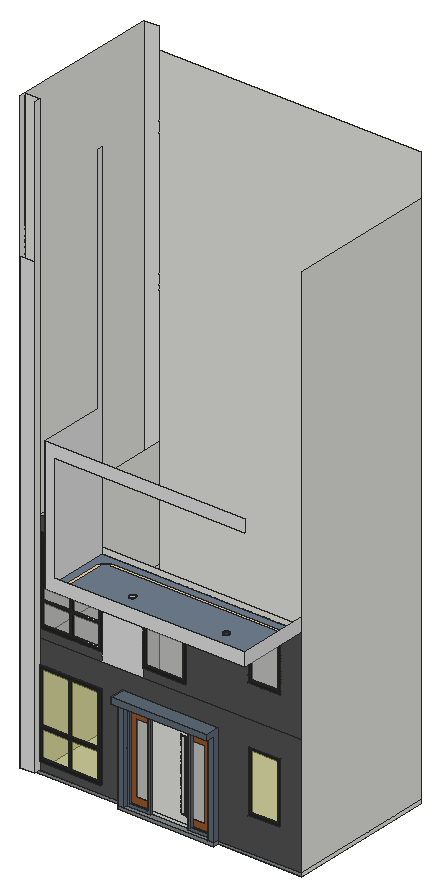
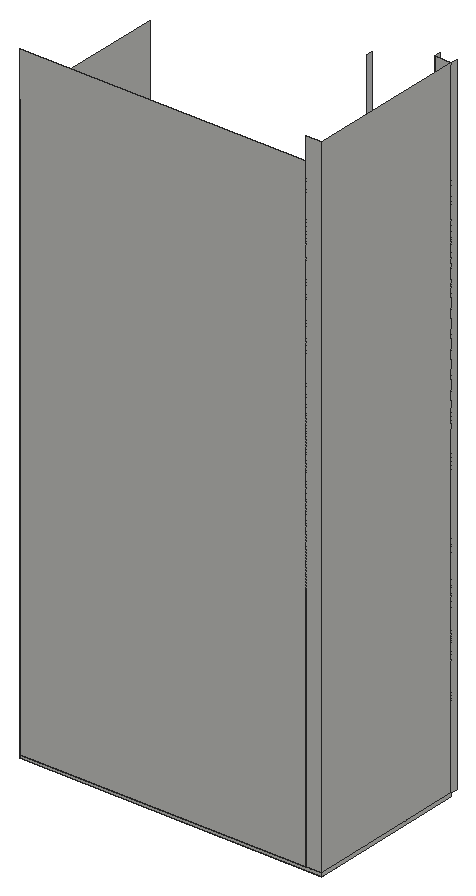
# SketchUp Ruby script. Lengths in inches.
U = 1.inch
M = Sketchup.active_model
def pt(a) = Geom::Point3d.new(a.map { |v| v * U })
def face(e, loops, mat)
  f = e.add_face(loops[0].map { |a| pt(a) })
  loops[1..].each { |l| e.add_face(l.map { |a| pt(a) }).erase! }
  f.material = f.back_material = mat if mat
  f
end
# faces: each face lists its corners as indices into pts; further lists are holes
def faces(e, pts, list, mat = nil) = list.each { |f| face(e, (f[0].is_a?(Array) ? f : [f]).map { |l| l.map { |i| pts[i] } }, mat) }
# xy, xz, yz: faces in a plane at the given z, y or x. An outline is a flat list of corners, or four numbers for a rectangle; further outlines are holes
def ring(l) = l.size == 4 ? [[l[0], l[1]], [l[2], l[1]], [l[2], l[3]], [l[0], l[3]]] : l.each_slice(2).to_a
def flat(e, list, mat, &to3) = list.each { |f| face(e, (f[0].is_a?(Array) ? f : [f]).map { |l| ring(l).map { |u, v| to3.(u, v) } }, mat) }
def xy(e, z, list, mat = nil) = flat(e, list, mat) { |x, y| [x, y, z] }
def xz(e, y, list, mat = nil) = flat(e, list, mat) { |x, z| [x, y, z] }
def yz(e, x, list, mat = nil) = flat(e, list, mat) { |y, z| [x, y, z] }
def lines(e, pts, list) = list.each { |a, b| e.add_line(pt(pts[a]), pt(pts[b])) }
# prism: a flat outline (further loops are holes) pulled along v
def prism(e, loops, v, mat = nil)
  f = face(e, loops, mat); d = Geom::Vector3d.new(v.map { |x| x * U })
  f.pushpull(f.normal.samedirection?(d) ? d.length : -d.length)
end
def box(e, o, s, mat = nil) = prism(e, [[o, [o[0] + s[0], o[1], o[2]], [o[0] + s[0], o[1] + s[1], o[2]], [o[0], o[1] + s[1], o[2]]]], [0, 0, s[2]], mat)
def at(x, y, z, deg = 0) = Geom::Transformation.translation(pt([x, y, z])) * Geom::Transformation.rotation(ORIGIN, Z_AXIS, deg.degrees)
def axes(o, x, y, z) = Geom::Transformation.new([*x, 0, *y, 0, *z, 0, *pt(o).to_a, 1])
def part(name) = M.definitions.add(name)
# library, detail: a bought-in or finely detailed component or shape, given as its bounding box
def library(name, o, s) = part(name).tap { |d| box(d.entities, o, s) }
def detail(e, o, s) = box(e.add_group.entities, o, s)
def put(e, d, t, mat = nil) = e.add_instance(d, t).tap { |i| i.material = mat if mat }
def group(e, t, mat = nil) = e.add_group.tap { |g| g.transformation = t; g.material = mat if mat }.entities
root = M.entities
M.materials.add("[0033_NavajoWhite]1").color = [237, 206, 160]
M.materials.add("[0110_LightSlateGray]").color = [93, 106, 119]
M.materials.add("[0111_SlateGray]").color = [112, 128, 144]
M.materials.add("[0132_LightGray]").color = [102, 102, 102]
M.materials.add("[0136_Charcoal]").color = [35, 35, 35]
M.materials.add("[Blacktop Old 01]").color = [132, 136, 139]
M.materials.add("[Cladding Siding White]1").color = [224, 224, 224]
M.materials.add("[Cladding Siding White]2").color = [81, 81, 81]
M.materials.add("[Translucent Glass Gray]1").color = [163, 163, 163]
M.materials["[Translucent Glass Gray]1"].alpha = 0.5
M.materials.add("[Translucent Glass Gray]2").color = [204, 203, 94]
M.materials["[Translucent Glass Gray]2"].alpha = 0.5
M.materials.add("[Translucent Glass Gray]3").color = [130, 130, 130]
M.materials["[Translucent Glass Gray]3"].alpha = 0.5
M.materials.add("[Wood Cherry Original]").color = [152, 86, 42]
xy(root,0,[[396,264,396,288,0,288,0,888,1116,888,1116,288,780,288,780,264]])
xy(root,12,[[0,264,60,288],[396,264,416.85,288],[759.15,264,780,288],[416.85,281,511.85,288],[664.15,281,759.15,288],
  [0,288,60,888],[60,288,1116,888]])
xy(root,12,[[416.85,264,759.15,264,759.15,281,664.15,281,664.15,288,511.85,288,511.85,281,416.85,281]],"[Blacktop Old 01]")
xy(root,23,[[427.85,281,499.85,288],[676.15,281,748.15,288]],"[0110_LightSlateGray]")
xy(root,48,[[60,282,312,288]],"[0136_Charcoal]")
xy(root,59.16,[[634.86,288,648.92,294]])
xy(root,60,[[72,282,181,288],[191,282,300,288]],"[0136_Charcoal]")
xy(root,156,[[912,288,1020,294]],"[0136_Charcoal]")
xy(root,168,[[72,282,181,288],[191,282,300,288]],"[0136_Charcoal]")
xy(root,180,[[72,282,181,288],[191,282,300,288]],"[0136_Charcoal]")
xy(root,338.39,[[634.86,288,648.92,294]])
xy(root,364.15,[[427.85,281,499.85,288],[511.85,281,664.15,288],[676.15,281,748.15,288]],"[0110_LightSlateGray]")
xy(root,375.15,[[416.85,281,759.15,288]])
xy(root,375.15,[[416.85,264,759.15,281]],"[0110_LightSlateGray]")
xy(root,384,[[181,282,191,288]])
xy(root,384,[[72,282,181,288],[191,282,300,288],[912,288,1020,294]],"[0136_Charcoal]")
xy(root,396,[[396,228,780,264]],"[0110_LightSlateGray]")
xy(root,396,[[60,282,312,288]],"[0136_Charcoal]")
xy(root,420,[[396,228,780,288]],"[0110_LightSlateGray]")
xy(root,540,[[72,288,181,295],[191,288,300,295]])
xy(root,540,[[487.9375,288,636,294]],"[0136_Charcoal]")
xy(root,624,[[72,288,181,295],[191,288,300,295]],"[0136_Charcoal]")
xy(root,630,[[72,288,181,295],[191,288,300,295]])
xy(root,636,[[912,288,1020,294]],"[0136_Charcoal]")
xy(root,864,[[72,288,181,295],[191,288,300,295],[487.9375,288,636,294],[912,288,1020,294]],"[0136_Charcoal]")
xy(root,882.9375,[[[385.0625,34.5,380.03,34.83,375.08,35.8125,370.3,37.43,365.78,39.67,361.59,42.47,357.79,45.79,354.47,49.59,351.67,53.78,349.43,58.3,347.8125,63.08,346.83,68.03,346.5,73.0625,346.5,214.9375,346.83,219.97,347.8125,224.92,349.43,229.7,351.67,234.22,354.47,238.41,357.79,242.21,361.59,245.53,365.78,248.33,370.3,250.57,375.08,252.1875,380.03,253.17,385.0625,253.5,1042.9375,253.5,1047.97,253.17,1052.92,252.1875,1057.7,250.57,1062.22,248.33,1066.41,245.53,1070.21,242.21,1073.53,238.41,1076.33,234.22,1078.57,229.7,1080.1875,224.92,1081.17,219.97,1081.5,214.9375,1081.5,73.0625,1081.17,68.03,1080.1875,63.08,1078.57,58.3,1076.33,53.78,1073.53,49.59,1070.21,45.79,1066.41,42.47,1062.22,39.67,1057.7,37.43,1052.92,35.8125,1047.97,34.83,1042.9375,34.5],[385.0625,40.83,1042.9375,40.83,1047.15,41.11,1051.28,41.93,1055.27,43.29,1059.05,45.15,1062.56,47.49,1065.73,50.27,1068.51,53.44,1070.85,56.95,1072.71,60.73,1074.07,64.72,1074.89,68.85,1075.17,73.0625,1075.17,214.9375,1074.89,219.15,1074.07,223.28,1072.71,227.27,1070.85,231.05,1068.51,234.56,1065.73,237.73,1062.56,240.51,1059.05,242.85,1055.27,244.71,1051.28,246.07,1047.15,246.89,1042.9375,247.17,385.0625,247.17,380.85,246.89,376.72,246.07,372.73,244.71,368.95,242.85,365.44,240.51,362.27,237.73,359.49,234.56,357.15,231.05,355.29,227.27,353.93,223.28,353.11,219.15,352.83,214.9375,352.83,73.0625,353.11,68.85,353.93,64.72,355.29,60.73,357.15,56.95,359.49,53.44,362.27,50.27,365.44,47.49,368.95,45.15,372.73,43.29,376.72,41.93,380.85,41.11]]],"[0033_NavajoWhite]1")
xy(root,882.9375,[[[312,0,1116,288],[385.0625,34.5,1042.9375,34.5,1047.97,34.83,1052.92,35.8125,1057.7,37.43,1062.22,39.67,1066.41,42.47,1070.21,45.79,1073.53,49.59,1076.33,53.78,1078.57,58.3,1080.1875,63.08,1081.17,68.03,1081.5,73.0625,1081.5,214.9375,1081.17,219.97,1080.1875,224.92,1078.57,229.7,1076.33,234.22,1073.53,238.41,1070.21,242.21,1066.41,245.53,1062.22,248.33,1057.7,250.57,1052.92,252.1875,1047.97,253.17,1042.9375,253.5,385.0625,253.5,380.03,253.17,375.08,252.1875,370.3,250.57,365.78,248.33,361.59,245.53,357.79,242.21,354.47,238.41,351.67,234.22,349.43,229.7,347.8125,224.92,346.83,219.97,346.5,214.9375,346.5,73.0625,346.83,68.03,347.8125,63.08,349.43,58.3,351.67,53.78,354.47,49.59,357.79,45.79,361.59,42.47,365.78,39.67,370.3,37.43,375.08,35.8125,380.03,34.83]],[[385.0625,40.83,380.85,41.11,376.72,41.93,372.73,43.29,368.95,45.15,365.44,47.49,362.27,50.27,359.49,53.44,357.15,56.95,355.29,60.73,353.93,64.72,353.11,68.85,352.83,73.0625,352.83,214.9375,353.11,219.15,353.93,223.28,355.29,227.27,357.15,231.05,359.49,234.56,362.27,237.73,365.44,240.51,368.95,242.85,372.73,244.71,376.72,246.07,380.85,246.89,385.0625,247.17,1042.9375,247.17,1047.15,246.89,1051.28,246.07,1055.27,244.71,1059.05,242.85,1062.56,240.51,1065.73,237.73,1068.51,234.56,1070.85,231.05,1072.71,227.27,1074.07,223.28,1074.89,219.15,1075.17,214.9375,1075.17,73.0625,1074.89,68.85,1074.07,64.72,1072.71,60.73,1070.85,56.95,1068.51,53.44,1065.73,50.27,1062.56,47.49,1059.05,45.15,1055.27,43.29,1051.28,41.93,1047.15,41.11,1042.9375,40.83],[559.63,120.38,560.88,120.5,562.11,120.75,563.31,121.13,564.46,121.63,565.55,122.25,566.57,122.98,567.51,123.82,568.36,124.74,569.11,125.76,569.74,126.84,570.26,127.98,570.66,129.17,570.93,130.4,571.07,131.65,571.08,132.9,570.96,134.15,570.71,135.39,570.33,136.58,569.82,137.73,569.2,138.83,568.47,139.85,567.64,140.79,566.71,141.64,565.7,142.38,564.62,143.02,563.48,143.54,562.28,143.93,561.06,144.2,559.81,144.35,558.55,144.35,557.3,144.23,556.07,143.98,554.875,143.6,553.72,143.1,552.63,142.48,551.61,141.75,550.67,140.92,549.82,139.99,549.08,138.98,548.44,137.9,547.92,136.75,547.52,135.56,547.25,134.33,547.11,133.09,547.1,131.83,547.23,130.58,547.48,129.35,547.86,128.15,548.36,127,548.98,125.91,549.71,124.89,550.54,123.95,551.47,123.1,552.48,122.35,553.5625,121.72,554.71,121.2,555.9,120.8,557.125,120.53,558.375,120.39],[937.5,120.38,938.75,120.5,939.98,120.75,941.18,121.13,942.33,121.63,943.43,122.25,944.45,122.98,945.39,123.82,946.24,124.74,946.98,125.76,947.62,126.84,948.14,127.98,948.53,129.17,948.8,130.4,948.95,131.65,948.95,132.9,948.83,134.15,948.58,135.39,948.2,136.58,947.7,137.73,947.08,138.83,946.35,139.85,945.52,140.79,944.59,141.64,943.58,142.38,942.5,143.02,941.35,143.54,940.16,143.93,938.93,144.2,937.69,144.35,936.43,144.35,935.18,144.23,933.95,143.98,932.75,143.6,931.6,143.1,930.51,142.48,929.49,141.75,928.55,140.92,927.7,139.99,926.95,138.98,926.32,137.9,925.8,136.75,925.4,135.56,925.13,134.33,924.99,133.09,924.98,131.83,925.1,130.58,925.35,129.35,925.73,128.15,926.23,127,926.85,125.91,927.58,124.89,928.42,123.95,929.34,123.1,930.36,122.35,931.4375,121.72,932.58,121.2,933.77,120.8,935,120.53,936.25,120.39]]],"[0111_SlateGray]")
xz(root,0,[[312,882.9375,1116,882.9375,1116,936,348,936,348,1366.34,1116,1366.34,1116,1416,312,1416]],"[Cladding Siding White]1")
xz(root,144.35,[[558.55,882.9375,559.81,883.9375],[936.43,882.9375,937.69,883.9375]])
xz(root,228,[[396,396,780,420]],"[0110_LightSlateGray]")
xz(root,264,[[396,12,416.85,12,416.85,375.15,759.15,375.15,759.15,12,780,12,780,396,396,396]],"[0110_LightSlateGray]")
xz(root,264,[[396,0,780,12]],"[Blacktop Old 01]")
xz(root,264,[[0,12,60,1858.15]],"[Cladding Siding White]1")
xz(root,281,[[[416.85,12,511.85,12,511.85,364.15,664.15,364.15,664.15,12,759.15,12,759.15,375.15,416.85,375.15],[427.85,23,499.85,364.15],[676.15,23,748.15,364.15]]],"[0110_LightSlateGray]")
xz(root,282,[[[60,48,312,396],[72,180,72,384,300,384,300,180,191,180,191,384,181,384,181,180],[191,60,300,168],[72,60,181,168]]],"[0136_Charcoal]")
xz(root,288,[[0,12,60,2436],[396,12,396,396,780,396,780,12,759.15,12,759.15,375.15,416.85,375.15,416.85,12],[[416.85,12,416.85,375.15,759.15,375.15,759.15,12,664.15,12,664.15,364.15,511.85,364.15,511.85,12],[427.85,23,499.85,364.15],[676.15,23,748.15,364.15]],[511.85,12,664.15,23],[[511.85,23,664.15,364.15],[628.7,53,655.08,344.55]],
  [[60,48,312,396],[72,180,181,180,181,384,191,384,191,180,300,180,300,384,72,384],[191,60,300,168],[72,60,181,168]],[312,882.9375,1116,906]])
xz(root,288,[[[628.7,53,655.08,344.55],[634.86,59.16,648.92,338.39]]],"[0132_LightGray]")
xz(root,288,[[[900,144,1032,396],[912,156,1020,384]],[[60,528,312,876],[191,630,300,864],[72,630,181,864],[72,540,181,624],[191,540,300,624]],[[475.9375,528,648,876],[487.9375,540,636,864]],[[900,624,1032,876],[912,636,1020,864]]],"[0136_Charcoal]")
xz(root,288,[[0,0,396,12],[780,0,1116,12]],"[Blacktop Old 01]")
xz(root,288,[[312,492,475.9375,882.9375]],"[Cladding Siding White]1")
xz(root,288,[[[60,12,396,12,396,420,780,420,780,12,1116,12,1116,492,60,492,60,396,312,396,312,48,60,48],[900,144,1032,396]],[60,492,312,528],[[475.9375,492,1116,492,1116,882.9375,475.9375,882.9375,475.9375,876,648,876,648,528,475.9375,528],[900,624,1032,876]],[60,876,312,936]],"[Cladding Siding White]2")
xz(root,288,[[72,60,181,168],[191,60,300,168],[72,180,181,384],[191,180,300,384]],"[Translucent Glass Gray]2")
xz(root,288,[[451.85,53,499.85,334.15],[676.15,53,724.15,334.15]],"[Translucent Glass Gray]3")
xz(root,288,[[427.85,23,499.85,23,499.85,53,451.85,53,451.85,334.15,499.85,334.15,499.85,364.15,427.85,364.15],[676.15,23,748.15,23,748.15,364.15,676.15,364.15,676.15,334.15,724.15,334.15,724.15,53,676.15,53]],"[Wood Cherry Original]")
xz(root,294,[[634.86,59.16,648.92,338.39]],"[0132_LightGray]")
xz(root,294,[[487.9375,540,636,864],[912,636,1020,864]],"[Translucent Glass Gray]1")
xz(root,294,[[912,156,1020,384]],"[Translucent Glass Gray]2")
xz(root,295,[[72,540,181,624],[191,540,300,624],[72,630,181,864],[191,630,300,864]],"[Translucent Glass Gray]1")
xz(root,888,[[0,0,1116,12],[0,12,60,2436],[60,12,1116,2352]])
yz(root,0,[[288,0,888,12],[264,12,288,2436],[288,12,888,2436]])
yz(root,60,[[264,12,288,12,288,48,282,48,282,396,288,396,288,2436,264,2436],[288,12,888,492],[282,48,288,396],[288,492,888,936]])
yz(root,72,[[282,60,288,168],[282,180,288,384],[288,540,295,624],[288,630,295,864]],"[0136_Charcoal]")
yz(root,181,[[288,540,295,624],[288,630,295,864]])
yz(root,181,[[282,60,288,168],[282,180,288,384]],"[0136_Charcoal]")
yz(root,191,[[282,60,288,168],[282,180,288,384],[288,540,295,624],[288,630,295,864]],"[0136_Charcoal]")
yz(root,300,[[282,60,288,168],[282,180,288,384],[288,540,295,624],[288,630,295,864]],"[0136_Charcoal]")
yz(root,312,[[282,48,288,396]],"[0136_Charcoal]")
yz(root,312,[[0,882.9375,0,1416,264,1416,264,2352,288,2352,288,882.9375]],"[Cladding Siding White]1")
yz(root,396,[[264,12,264,396,228,396,228,420,288,420,288,12]],"[0110_LightSlateGray]")
yz(root,396,[[264,0,288,12]],"[Blacktop Old 01]")
yz(root,416.85,[[281,12,288,375.15]])
yz(root,416.85,[[264,12,281,375.15]],"[0110_LightSlateGray]")
yz(root,427.85,[[281,23,288,364.15]],"[0110_LightSlateGray]")
yz(root,487.9375,[[288,540,294,864]],"[0136_Charcoal]")
yz(root,499.85,[[281,23,288,364.15]],"[0110_LightSlateGray]")
yz(root,511.85,[[281,12,288,364.15]],"[0110_LightSlateGray]")
yz(root,634.86,[[288,59.16,294,338.39]])
yz(root,636,[[288,540,294,864]],"[0136_Charcoal]")
yz(root,648.92,[[288,59.16,294,338.39]])
yz(root,664.15,[[281,12,288,364.15]],"[0110_LightSlateGray]")
yz(root,676.15,[[281,23,288,364.15]],"[0110_LightSlateGray]")
yz(root,748.15,[[281,23,288,364.15]],"[0110_LightSlateGray]")
yz(root,759.15,[[281,12,288,375.15]])
yz(root,759.15,[[264,12,281,375.15]],"[0110_LightSlateGray]")
yz(root,780,[[264,12,288,12,288,420,228,420,228,396,264,396]],"[0110_LightSlateGray]")
yz(root,780,[[264,0,288,12]],"[Blacktop Old 01]")
yz(root,912,[[288,156,294,384],[288,636,294,864]],"[0136_Charcoal]")
yz(root,948.95,[[131.65,882.9375,132.9,883.9375]])
yz(root,1020,[[288,156,294,384],[288,636,294,864]],"[0136_Charcoal]")
yz(root,1116,[[288,0,888,12],[288,12,888,2184]])
yz(root,1116,[[0,882.9375,288,936]],"[Cladding Siding White]1")
p = [[558.375,120.39,882.9375],[557.125,120.53,882.9375],[557.125,120.53,883.9375],[558.375,120.39,883.9375],[559.63,120.38,882.9375],[559.63,120.38,883.9375],
  [560.88,120.5,882.9375],[560.88,120.5,883.9375],[936.25,120.39,882.9375],[935,120.53,882.9375],[935,120.53,883.9375],[936.25,120.39,883.9375],
  [937.5,120.38,882.9375],[937.5,120.38,883.9375],[938.75,120.5,882.9375],[938.75,120.5,883.9375],[555.9,120.8,882.9375],[555.9,120.8,883.9375],
  [562.11,120.75,882.9375],[562.11,120.75,883.9375],[933.77,120.8,882.9375],[933.77,120.8,883.9375],[939.98,120.75,882.9375],[939.98,120.75,883.9375],
  [554.71,121.2,882.9375],[554.71,121.2,883.9375],[563.31,121.13,882.9375],[563.31,121.13,883.9375],[932.58,121.2,882.9375],[932.58,121.2,883.9375],
  [941.18,121.13,882.9375],[941.18,121.13,883.9375],[564.46,121.63,882.9375],[564.46,121.63,883.9375],[942.33,121.63,882.9375],[942.33,121.63,883.9375],
  [553.5625,121.72,882.9375],[553.5625,121.72,883.9375],[931.4375,121.72,882.9375],[931.4375,121.72,883.9375],[565.55,122.25,882.9375],[565.55,122.25,883.9375],
  [943.43,122.25,882.9375],[943.43,122.25,883.9375],[552.48,122.35,882.9375],[552.48,122.35,883.9375],[930.36,122.35,882.9375],[930.36,122.35,883.9375],
  [566.57,122.98,882.9375],[566.57,122.98,883.9375],[944.45,122.98,882.9375],[944.45,122.98,883.9375],[551.47,123.1,882.9375],[551.47,123.1,883.9375],
  [929.34,123.1,882.9375],[929.34,123.1,883.9375],[567.51,123.82,882.9375],[567.51,123.82,883.9375],[945.39,123.82,882.9375],[945.39,123.82,883.9375],
  [550.54,123.95,882.9375],[550.54,123.95,883.9375],[928.42,123.95,882.9375],[928.42,123.95,883.9375],[568.36,124.74,882.9375],[568.36,124.74,883.9375],
  [946.24,124.74,882.9375],[946.24,124.74,883.9375],[549.71,124.89,882.9375],[549.71,124.89,883.9375],[927.58,124.89,882.9375],[927.58,124.89,883.9375],
  [569.11,125.76,882.9375],[569.11,125.76,883.9375],[946.98,125.76,882.9375],[946.98,125.76,883.9375],[548.98,125.91,882.9375],[548.98,125.91,883.9375],
  [926.85,125.91,882.9375],[926.85,125.91,883.9375],[569.74,126.84,882.9375],[569.74,126.84,883.9375],[947.62,126.84,882.9375],[947.62,126.84,883.9375],
  [548.36,127,882.9375],[548.36,127,883.9375],[926.23,127,882.9375],[926.23,127,883.9375],[570.26,127.98,882.9375],[570.26,127.98,883.9375],
  [948.14,127.98,882.9375],[948.14,127.98,883.9375],[547.86,128.15,882.9375],[547.86,128.15,883.9375],[925.73,128.15,882.9375],[925.73,128.15,883.9375],
  [570.66,129.17,882.9375],[570.66,129.17,883.9375],[948.53,129.17,882.9375],[948.53,129.17,883.9375],[547.48,129.35,882.9375],[547.48,129.35,883.9375],
  [925.35,129.35,882.9375],[925.35,129.35,883.9375],[570.93,130.4,882.9375],[570.93,130.4,883.9375],[948.8,130.4,882.9375],[948.8,130.4,883.9375],
  [547.23,130.58,882.9375],[547.23,130.58,883.9375],[925.1,130.58,882.9375],[925.1,130.58,883.9375],[571.07,131.65,882.9375],[571.07,131.65,883.9375],
  [948.95,131.65,882.9375],[948.95,131.65,883.9375],[547.1,131.83,882.9375],[547.1,131.83,883.9375],[924.98,131.83,882.9375],[924.98,131.83,883.9375],
  [571.08,132.9,882.9375],[571.08,132.9,883.9375],[547.11,133.09,882.9375],[547.11,133.09,883.9375],[924.99,133.09,882.9375],[924.99,133.09,883.9375],
  [570.96,134.15,882.9375],[570.96,134.15,883.9375],[948.83,134.15,882.9375],[948.95,132.9,882.9375],[948.95,132.9,883.9375],[948.83,134.15,883.9375],
  [547.25,134.33,882.9375],[547.25,134.33,883.9375],[925.13,134.33,882.9375],[925.13,134.33,883.9375],[570.71,135.39,882.9375],[570.71,135.39,883.9375],
  [948.58,135.39,882.9375],[948.58,135.39,883.9375],[547.52,135.56,882.9375],[547.52,135.56,883.9375],[925.4,135.56,882.9375],[925.4,135.56,883.9375],
  [570.33,136.58,882.9375],[570.33,136.58,883.9375],[948.2,136.58,882.9375],[948.2,136.58,883.9375],[547.92,136.75,882.9375],[547.92,136.75,883.9375],
  [925.8,136.75,882.9375],[925.8,136.75,883.9375],[569.82,137.73,882.9375],[569.82,137.73,883.9375],[947.7,137.73,882.9375],[947.7,137.73,883.9375],
  [548.44,137.9,882.9375],[548.44,137.9,883.9375],[926.32,137.9,882.9375],[926.32,137.9,883.9375],[569.2,138.83,882.9375],[569.2,138.83,883.9375],
  [947.08,138.83,882.9375],[947.08,138.83,883.9375],[549.08,138.98,882.9375],[549.08,138.98,883.9375],[926.95,138.98,882.9375],[926.95,138.98,883.9375],
  [568.47,139.85,882.9375],[568.47,139.85,883.9375],[946.35,139.85,882.9375],[946.35,139.85,883.9375],[549.82,139.99,882.9375],[549.82,139.99,883.9375],
  [927.7,139.99,882.9375],[927.7,139.99,883.9375],[567.64,140.79,882.9375],[567.64,140.79,883.9375],[945.52,140.79,882.9375],[945.52,140.79,883.9375],
  [550.67,140.92,882.9375],[550.67,140.92,883.9375],[928.55,140.92,882.9375],[928.55,140.92,883.9375],[566.71,141.64,882.9375],[566.71,141.64,883.9375],
  [944.59,141.64,882.9375],[944.59,141.64,883.9375],[551.61,141.75,882.9375],[551.61,141.75,883.9375],[929.49,141.75,882.9375],[929.49,141.75,883.9375],
  [565.7,142.38,882.9375],[565.7,142.38,883.9375],[943.58,142.38,882.9375],[943.58,142.38,883.9375],[552.63,142.48,882.9375],[552.63,142.48,883.9375],
  [930.51,142.48,882.9375],[930.51,142.48,883.9375],[564.62,143.02,882.9375],[564.62,143.02,883.9375],[942.5,143.02,882.9375],[942.5,143.02,883.9375],
  [553.72,143.1,882.9375],[553.72,143.1,883.9375],[931.6,143.1,882.9375],[931.6,143.1,883.9375],[563.48,143.54,882.9375],[563.48,143.54,883.9375],
  [941.35,143.54,882.9375],[941.35,143.54,883.9375],[554.875,143.6,882.9375],[554.875,143.6,883.9375],[932.75,143.6,882.9375],[932.75,143.6,883.9375],
  [562.28,143.93,882.9375],[562.28,143.93,883.9375],[940.16,143.93,882.9375],[940.16,143.93,883.9375],[556.07,143.98,882.9375],[556.07,143.98,883.9375],
  [933.95,143.98,882.9375],[933.95,143.98,883.9375],[561.06,144.2,882.9375],[561.06,144.2,883.9375],[938.93,144.2,882.9375],[938.93,144.2,883.9375],
  [557.3,144.23,882.9375],[557.3,144.23,883.9375],[935.18,144.23,882.9375],[935.18,144.23,883.9375],[558.55,144.35,882.9375],[558.55,144.35,883.9375],
  [559.81,144.35,882.9375],[559.81,144.35,883.9375],[936.43,144.35,882.9375],[936.43,144.35,883.9375],[937.69,144.35,882.9375],[937.69,144.35,883.9375]]
faces(root,p,[[0,1,2,3],[4,0,3,5],[6,4,5,7],[8,9,10,11],[12,8,11,13],[14,12,13,15],[1,16,17,2],[18,6,7,19],
  [9,20,21,10],[22,14,15,23],[16,24,25,17],[26,18,19,27],[20,28,29,21],[30,22,23,31],[32,26,27,33],[34,30,31,35],
  [24,36,37,25],[28,38,39,29],[40,32,33,41],[42,34,35,43],[36,44,45,37],[38,46,47,39],[48,40,41,49],[50,42,43,51],
  [44,52,53,45],[46,54,55,47],[56,48,49,57],[58,50,51,59],[52,60,61,53],[54,62,63,55],[64,56,57,65],[66,58,59,67],
  [60,68,69,61],[62,70,71,63],[72,64,65,73],[74,66,67,75],[68,76,77,69],[70,78,79,71],[80,72,73,81],[82,74,75,83],
  [76,84,85,77],[78,86,87,79],[88,80,81,89],[90,82,83,91],[84,92,93,85],[86,94,95,87],[96,88,89,97],[98,90,91,99],
  [92,100,101,93],[94,102,103,95],[104,96,97,105],[106,98,99,107],[100,108,109,101],[102,110,111,103],[112,104,105,113],[114,106,107,115],
  [108,116,117,109],[110,118,119,111],[120,112,113,121],[116,122,123,117],[118,124,125,119],[126,120,121,127],[128,129,130,131],[122,132,133,123],
  [124,134,135,125],[136,126,127,137],[138,128,131,139],[132,140,141,133],[134,142,143,135],[144,136,137,145],[146,138,139,147],[140,148,149,141],
  [142,150,151,143],[152,144,145,153],[154,146,147,155],[148,156,157,149],[150,158,159,151],[160,152,153,161],[162,154,155,163],[156,164,165,157],
  [158,166,167,159],[168,160,161,169],[170,162,163,171],[164,172,173,165],[166,174,175,167],[176,168,169,177],[178,170,171,179],[172,180,181,173],
  [174,182,183,175],[184,176,177,185],[186,178,179,187],[180,188,189,181],[182,190,191,183],[192,184,185,193],[194,186,187,195],[188,196,197,189],
  [190,198,199,191],[200,192,193,201],[202,194,195,203],[196,204,205,197],[198,206,207,199],[208,200,201,209],[210,202,203,211],[204,212,213,205],
  [206,214,215,207],[216,208,209,217],[218,210,211,219],[212,220,221,213],[214,222,223,215],[224,216,217,225],[226,218,219,227],[220,228,229,221],
  [222,230,231,223],[228,232,233,229],[234,224,225,235],[230,236,237,231],[238,226,227,239]])
